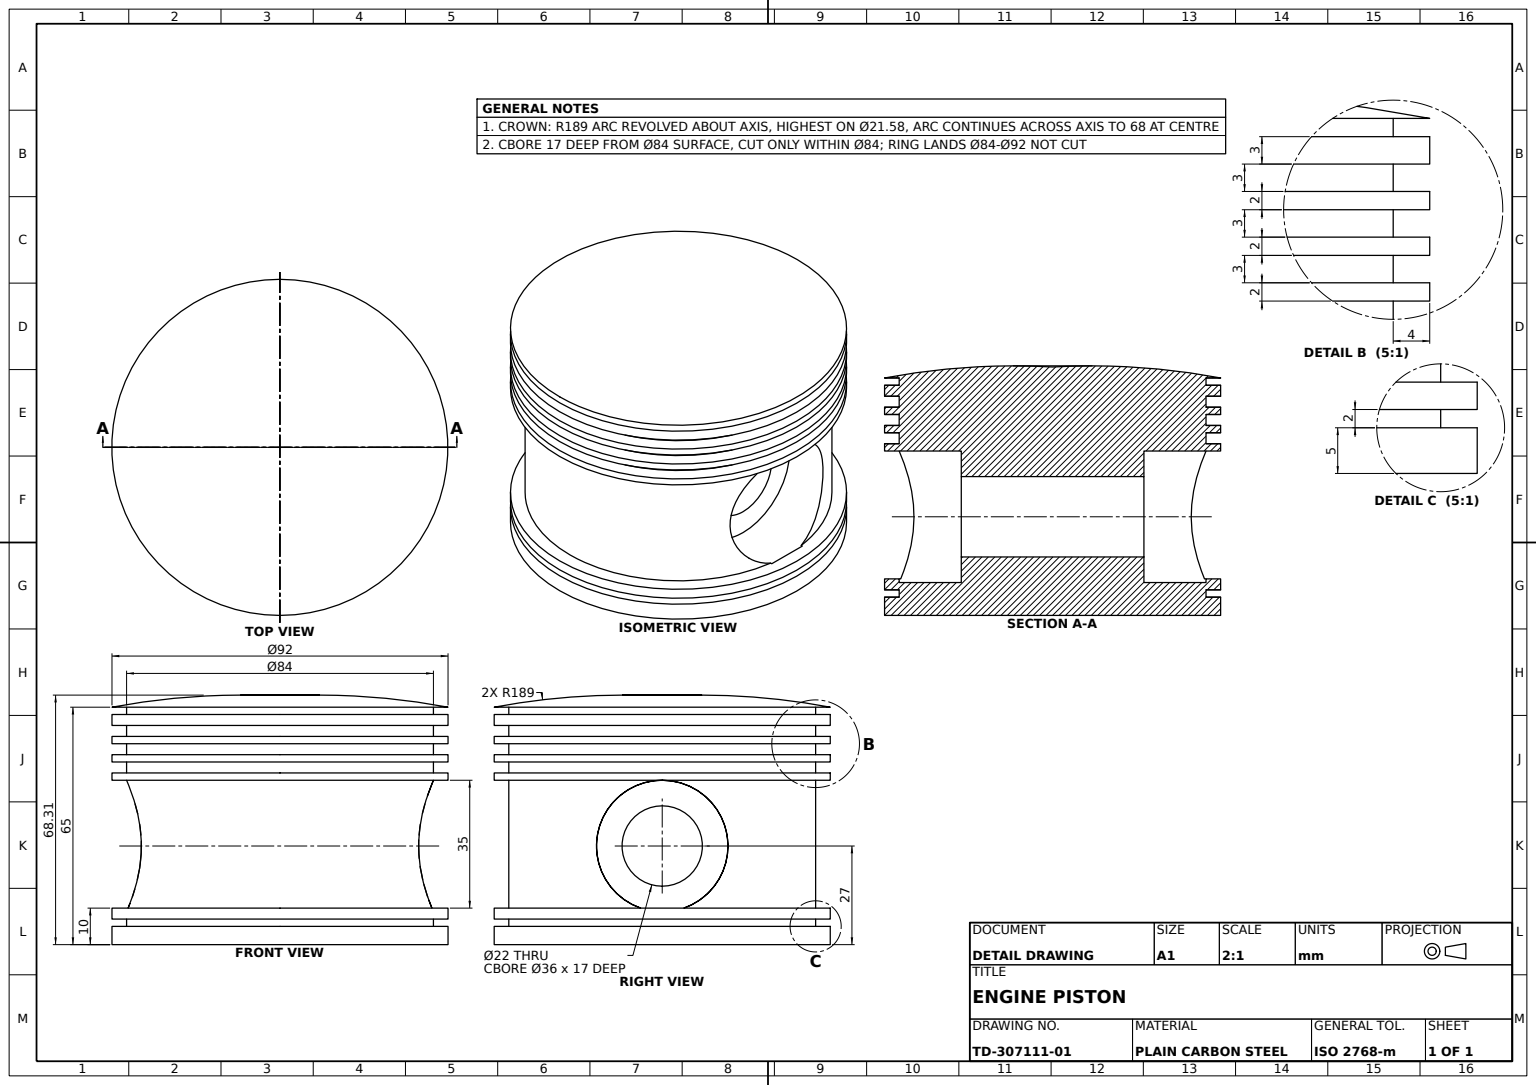
ISO-10303-21;
HEADER;
FILE_DESCRIPTION((''),'2;1');
FILE_NAME('','',(''),(''),'','','');
FILE_SCHEMA(('AUTOMOTIVE_DESIGN'));
ENDSEC;
DATA;
#1=APPLICATION_CONTEXT('');
#2=PRODUCT_CONTEXT('',#1,'mechanical');
#3=PRODUCT('','','',(#2));
#4=PRODUCT_DEFINITION_FORMATION('','',#3);
#5=PRODUCT_DEFINITION_CONTEXT('',#1,'design');
#6=PRODUCT_DEFINITION('','',#4,#5);
#7=PRODUCT_DEFINITION_SHAPE('','',#6);
#8=(LENGTH_UNIT()NAMED_UNIT(*)SI_UNIT(.MILLI.,.METRE.));
#9=(NAMED_UNIT(*)PLANE_ANGLE_UNIT()SI_UNIT($,.RADIAN.));
#10=(NAMED_UNIT(*)SI_UNIT($,.STERADIAN.)SOLID_ANGLE_UNIT());
#11=UNCERTAINTY_MEASURE_WITH_UNIT(LENGTH_MEASURE(1.E-05),#8,'distance_accuracy_value','');
#12=(GEOMETRIC_REPRESENTATION_CONTEXT(3)GLOBAL_UNCERTAINTY_ASSIGNED_CONTEXT((#11))GLOBAL_UNIT_ASSIGNED_CONTEXT((#8,#9,#10))REPRESENTATION_CONTEXT('',''));
#13=CARTESIAN_POINT('',(-46.,0.,-47.));
#14=VERTEX_POINT('',#13);
#15=CARTESIAN_POINT('',(-46.,0.,-45.));
#16=VERTEX_POINT('',#15);
#17=CARTESIAN_POINT('',(-46.,0.,0.));
#18=DIRECTION('',(0.,0.,1.));
#19=VECTOR('',#18,1000.);
#20=LINE('',#17,#19);
#21=EDGE_CURVE('',#14,#16,#20,.T.);
#22=ORIENTED_EDGE('',*,*,#21,.F.);
#23=CARTESIAN_POINT('',(46.,0.,-47.));
#24=VERTEX_POINT('',#23);
#25=CARTESIAN_POINT('',(0.,0.,-47.));
#26=DIRECTION('',(1.,0.,0.));
#27=AXIS2_PLACEMENT_3D('',#25,#18,#26);
#28=CIRCLE('',#27,46.);
#29=EDGE_CURVE('',#14,#24,#28,.T.);
#30=ORIENTED_EDGE('',*,*,#29,.T.);
#31=CARTESIAN_POINT('',(46.,0.,-45.));
#32=VERTEX_POINT('',#31);
#33=CARTESIAN_POINT('',(46.,0.,0.));
#34=LINE('',#33,#19);
#35=EDGE_CURVE('',#24,#32,#34,.T.);
#36=ORIENTED_EDGE('',*,*,#35,.T.);
#37=CARTESIAN_POINT('',(0.,0.,-45.));
#38=AXIS2_PLACEMENT_3D('',#37,#18,#26);
#39=CIRCLE('',#38,46.);
#40=EDGE_CURVE('',#16,#32,#39,.T.);
#41=ORIENTED_EDGE('',*,*,#40,.F.);
#42=EDGE_LOOP('',(#22,#30,#36,#41));
#43=FACE_OUTER_BOUND('',#42,.T.);
#44=CARTESIAN_POINT('',(0.,0.,0.));
#45=AXIS2_PLACEMENT_3D('',#44,#18,#26);
#46=CYLINDRICAL_SURFACE('',#45,46.);
#47=ADVANCED_FACE('',(#43),#46,.T.);
#48=CARTESIAN_POINT('',(46.,0.,-50.));
#49=VERTEX_POINT('',#48);
#50=CARTESIAN_POINT('',(-46.,0.,-50.));
#51=VERTEX_POINT('',#50);
#52=CARTESIAN_POINT('',(0.,0.,-50.));
#53=AXIS2_PLACEMENT_3D('',#52,#18,#26);
#54=CIRCLE('',#53,46.);
#55=EDGE_CURVE('',#49,#51,#54,.T.);
#56=ORIENTED_EDGE('',*,*,#55,.F.);
#57=CARTESIAN_POINT('',(46.,0.,-52.));
#58=VERTEX_POINT('',#57);
#59=EDGE_CURVE('',#58,#49,#34,.T.);
#60=ORIENTED_EDGE('',*,*,#59,.F.);
#61=CARTESIAN_POINT('',(-46.,0.,-52.));
#62=VERTEX_POINT('',#61);
#63=CARTESIAN_POINT('',(0.,0.,-52.));
#64=AXIS2_PLACEMENT_3D('',#63,#18,#26);
#65=CIRCLE('',#64,46.);
#66=EDGE_CURVE('',#58,#62,#65,.T.);
#67=ORIENTED_EDGE('',*,*,#66,.T.);
#68=EDGE_CURVE('',#62,#51,#20,.T.);
#69=ORIENTED_EDGE('',*,*,#68,.T.);
#70=EDGE_LOOP('',(#56,#60,#67,#69));
#71=FACE_OUTER_BOUND('',#70,.T.);
#72=ADVANCED_FACE('',(#71),#46,.T.);
#73=ORIENTED_EDGE('',*,*,#21,.T.);
#74=EDGE_CURVE('',#32,#16,#39,.T.);
#75=ORIENTED_EDGE('',*,*,#74,.F.);
#76=ORIENTED_EDGE('',*,*,#35,.F.);
#77=EDGE_CURVE('',#24,#14,#28,.T.);
#78=ORIENTED_EDGE('',*,*,#77,.T.);
#79=EDGE_LOOP('',(#73,#75,#76,#78));
#80=FACE_OUTER_BOUND('',#79,.T.);
#81=ADVANCED_FACE('',(#80),#46,.T.);
#82=CARTESIAN_POINT('',(42.,0.,-5.));
#83=VERTEX_POINT('',#82);
#84=CARTESIAN_POINT('',(-42.,0.,-5.));
#85=VERTEX_POINT('',#84);
#86=CARTESIAN_POINT('',(0.,0.,-5.));
#87=AXIS2_PLACEMENT_3D('',#86,#18,#26);
#88=CIRCLE('',#87,42.);
#89=EDGE_CURVE('',#83,#85,#88,.T.);
#90=ORIENTED_EDGE('',*,*,#89,.F.);
#91=CARTESIAN_POINT('',(42.,0.,-7.));
#92=VERTEX_POINT('',#91);
#93=CARTESIAN_POINT('',(42.,0.,0.));
#94=LINE('',#93,#19);
#95=EDGE_CURVE('',#92,#83,#94,.T.);
#96=ORIENTED_EDGE('',*,*,#95,.F.);
#97=CARTESIAN_POINT('',(-42.,0.,-7.));
#98=VERTEX_POINT('',#97);
#99=CARTESIAN_POINT('',(0.,0.,-7.));
#100=AXIS2_PLACEMENT_3D('',#99,#18,#26);
#101=CIRCLE('',#100,42.);
#102=EDGE_CURVE('',#92,#98,#101,.T.);
#103=ORIENTED_EDGE('',*,*,#102,.T.);
#104=CARTESIAN_POINT('',(-42.,0.,0.));
#105=LINE('',#104,#19);
#106=EDGE_CURVE('',#98,#85,#105,.T.);
#107=ORIENTED_EDGE('',*,*,#106,.T.);
#108=EDGE_LOOP('',(#90,#96,#103,#107));
#109=FACE_OUTER_BOUND('',#108,.T.);
#110=CYLINDRICAL_SURFACE('',#45,42.);
#111=ADVANCED_FACE('',(#109),#110,.T.);
#112=ORIENTED_EDGE('',*,*,#102,.F.);
#113=EDGE_CURVE('',#98,#92,#101,.T.);
#114=ORIENTED_EDGE('',*,*,#113,.F.);
#115=EDGE_LOOP('',(#112,#114));
#116=FACE_BOUND('',#115,.T.);
#117=CARTESIAN_POINT('',(46.,0.,-7.));
#118=VERTEX_POINT('',#117);
#119=CARTESIAN_POINT('',(-46.,0.,-7.));
#120=VERTEX_POINT('',#119);
#121=CIRCLE('',#100,46.);
#122=EDGE_CURVE('',#118,#120,#121,.T.);
#123=ORIENTED_EDGE('',*,*,#122,.T.);
#124=EDGE_CURVE('',#120,#118,#121,.T.);
#125=ORIENTED_EDGE('',*,*,#124,.T.);
#126=EDGE_LOOP('',(#123,#125));
#127=FACE_OUTER_BOUND('',#126,.T.);
#128=PLANE('',#100);
#129=ADVANCED_FACE('',(#116,#127),#128,.T.);
#130=CARTESIAN_POINT('',(-42.,0.,-55.));
#131=VERTEX_POINT('',#130);
#132=CARTESIAN_POINT('',(42.,0.,-55.));
#133=VERTEX_POINT('',#132);
#134=CARTESIAN_POINT('',(0.,0.,-55.));
#135=AXIS2_PLACEMENT_3D('',#134,#18,#26);
#136=CIRCLE('',#135,42.);
#137=EDGE_CURVE('',#131,#133,#136,.T.);
#138=ORIENTED_EDGE('',*,*,#137,.T.);
#139=CARTESIAN_POINT('',(42.,0.,-52.));
#140=VERTEX_POINT('',#139);
#141=EDGE_CURVE('',#133,#140,#94,.T.);
#142=ORIENTED_EDGE('',*,*,#141,.T.);
#143=CARTESIAN_POINT('',(-42.,0.,-52.));
#144=VERTEX_POINT('',#143);
#145=CIRCLE('',#64,42.);
#146=EDGE_CURVE('',#144,#140,#145,.T.);
#147=ORIENTED_EDGE('',*,*,#146,.F.);
#148=EDGE_CURVE('',#131,#144,#105,.T.);
#149=ORIENTED_EDGE('',*,*,#148,.F.);
#150=EDGE_LOOP('',(#138,#142,#147,#149));
#151=FACE_OUTER_BOUND('',#150,.T.);
#152=ADVANCED_FACE('',(#151),#110,.T.);
#153=CARTESIAN_POINT('',(-5.91608,41.581246,-10.));
#154=VERTEX_POINT('',#153);
#155=CARTESIAN_POINT('',(-5.91608,42.,-10.));
#156=VERTEX_POINT('',#155);
#157=CARTESIAN_POINT('',(-5.91608,25.,-10.));
#158=DIRECTION('',(0.,1.,0.));
#159=VECTOR('',#158,1000.);
#160=LINE('',#157,#159);
#161=EDGE_CURVE('',#154,#156,#160,.T.);
#162=ORIENTED_EDGE('',*,*,#161,.T.);
#163=CARTESIAN_POINT('',(0.,42.,-9.));
#164=VERTEX_POINT('',#163);
#165=CARTESIAN_POINT('',(0.,42.,-27.));
#166=AXIS2_PLACEMENT_3D('',#165,#158,#18);
#167=CIRCLE('',#166,18.);
#168=EDGE_CURVE('',#156,#164,#167,.T.);
#169=ORIENTED_EDGE('',*,*,#168,.T.);
#170=CARTESIAN_POINT('',(0.,25.,-9.));
#171=VERTEX_POINT('',#170);
#172=LINE('',#170,#159);
#173=EDGE_CURVE('',#171,#164,#172,.T.);
#174=ORIENTED_EDGE('',*,*,#173,.F.);
#175=CARTESIAN_POINT('',(0.,25.,-45.));
#176=VERTEX_POINT('',#175);
#177=CARTESIAN_POINT('',(0.,25.,-27.));
#178=AXIS2_PLACEMENT_3D('',#177,#158,#18);
#179=CIRCLE('',#178,18.);
#180=EDGE_CURVE('',#176,#171,#179,.T.);
#181=ORIENTED_EDGE('',*,*,#180,.F.);
#182=CARTESIAN_POINT('',(0.,42.,-45.));
#183=VERTEX_POINT('',#182);
#184=LINE('',#175,#159);
#185=EDGE_CURVE('',#176,#183,#184,.T.);
#186=ORIENTED_EDGE('',*,*,#185,.T.);
#187=CARTESIAN_POINT('',(-1.061109,42.,-45.));
#188=CARTESIAN_POINT('',(-2.121977,41.95976,-44.906731));
#189=CARTESIAN_POINT('',(-4.236491,41.799239,-44.527291));
#190=CARTESIAN_POINT('',(-5.257741,41.68158,-44.24719));
#191=CARTESIAN_POINT('',(-6.739523,41.458754,-43.698988));
#192=CARTESIAN_POINT('',(-7.225049,41.376736,-43.494768));
#193=CARTESIAN_POINT('',(-8.179372,41.198707,-43.042961));
#194=CARTESIAN_POINT('',(-8.64942,41.10235,-42.794419));
#195=CARTESIAN_POINT('',(-10.009425,40.800416,-41.997198));
#196=CARTESIAN_POINT('',(-10.857804,40.580658,-41.394135));
#197=CARTESIAN_POINT('',(-12.047698,40.23709,-40.383712));
#198=CARTESIAN_POINT('',(-12.430461,40.120239,-40.029148));
#199=CARTESIAN_POINT('',(-13.167974,39.884262,-39.283303));
#200=CARTESIAN_POINT('',(-13.519453,39.766169,-38.895167));
#201=CARTESIAN_POINT('',(-14.516037,39.418016,-37.694253));
#202=CARTESIAN_POINT('',(-15.107299,39.192876,-36.841775));
#203=CARTESIAN_POINT('',(-15.885032,38.881149,-35.481657));
#204=CARTESIAN_POINT('',(-16.125966,38.781584,-35.014634));
#205=CARTESIAN_POINT('',(-16.569756,38.594057,-34.051546));
#206=CARTESIAN_POINT('',(-16.769263,38.507524,-33.562673));
#207=CARTESIAN_POINT('',(-17.30133,38.272892,-32.076551));
#208=CARTESIAN_POINT('',(-17.568459,38.149543,-31.058911));
#209=CARTESIAN_POINT('',(-17.83483,38.025366,-29.49002));
#210=CARTESIAN_POINT('',(-17.901168,37.994084,-28.959073));
#211=CARTESIAN_POINT('',(-17.98625,37.95388,-27.885782));
#212=CARTESIAN_POINT('',(-18.004438,37.945227,-27.35139));
#213=CARTESIAN_POINT('',(-17.988399,37.952835,-25.754766));
#214=CARTESIAN_POINT('',(-17.884108,38.002716,-24.699044));
#215=CARTESIAN_POINT('',(-17.586774,38.140757,-23.128397));
#216=CARTESIAN_POINT('',(-17.463221,38.19766,-22.604707));
#217=CARTESIAN_POINT('',(-17.173338,38.328863,-21.581592));
#218=CARTESIAN_POINT('',(-17.00688,38.403227,-21.080313));
#219=CARTESIAN_POINT('',(-16.444866,38.64885,-19.605884));
#220=CARTESIAN_POINT('',(-15.986987,38.842708,-18.661532));
#221=CARTESIAN_POINT('',(-14.902994,39.27137,-16.850389));
#222=CARTESIAN_POINT('',(-14.29136,39.500285,-16.007521));
#223=CARTESIAN_POINT('',(-13.27255,39.84932,-14.830004));
#224=CARTESIAN_POINT('',(-12.915936,39.966639,-14.45207));
#225=CARTESIAN_POINT('',(-12.167816,40.20072,-13.725355));
#226=CARTESIAN_POINT('',(-11.774245,40.318048,-13.374974));
#227=CARTESIAN_POINT('',(-10.556333,40.660487,-12.382869));
#228=CARTESIAN_POINT('',(-9.696644,40.875872,-11.799435));
#229=CARTESIAN_POINT('',(-7.881048,41.264403,-10.783615));
#230=CARTESIAN_POINT('',(-6.925197,41.437671,-10.351177));
#231=B_SPLINE_CURVE_WITH_KNOTS('',3,(#182,#187,#188,#189,#190,#191,#192,#193,#194,#195,#196,#197,#198,#199,#200,#201,#202,#203,#204,#205,#206,#207,#208,#209,#210,#211,#212,#213,#214,#215,#216,#217,#218,#219,#220,#221,#222,#223,#224,#225,#226,#227,#228,#229,#230,#153),.UNSPECIFIED.,.F.,.F.,(4,2,2,2,2,2,2,2,2,2,2,2,2,2,2,2,2,2,2,2,2,2,4),(0.050941496,0.05412348,0.057305464,0.058896456,0.060487448,0.063669432,0.065260424,0.066851416,0.0700334,0.071624392,0.073215384,0.076397368,0.07798836,0.079579352,0.082761336,0.084352328,0.08594332,0.089125304,0.092307288,0.09389828,0.095489272,0.098671256,0.10185324),.UNSPECIFIED.);
#232=EDGE_CURVE('',#183,#154,#231,.T.);
#233=ORIENTED_EDGE('',*,*,#232,.T.);
#234=EDGE_LOOP('',(#162,#169,#174,#181,#186,#233));
#235=FACE_OUTER_BOUND('',#234,.T.);
#236=CYLINDRICAL_SURFACE('',#178,18.);
#237=ADVANCED_FACE('',(#235),#236,.F.);
#238=CARTESIAN_POINT('',(5.91608,42.,-10.));
#239=VERTEX_POINT('',#238);
#240=CARTESIAN_POINT('',(0.,42.,-10.));
#241=VECTOR('',#26,1000.);
#242=LINE('',#240,#241);
#243=EDGE_CURVE('',#156,#239,#242,.T.);
#244=ORIENTED_EDGE('',*,*,#243,.T.);
#245=EDGE_CURVE('',#164,#239,#167,.T.);
#246=ORIENTED_EDGE('',*,*,#245,.F.);
#247=ORIENTED_EDGE('',*,*,#168,.F.);
#248=EDGE_LOOP('',(#244,#246,#247));
#249=FACE_OUTER_BOUND('',#248,.T.);
#250=PLANE('',#166);
#251=ADVANCED_FACE('',(#249),#250,.F.);
#252=ORIENTED_EDGE('',*,*,#77,.F.);
#253=ORIENTED_EDGE('',*,*,#29,.F.);
#254=EDGE_LOOP('',(#252,#253));
#255=FACE_OUTER_BOUND('',#254,.T.);
#256=CARTESIAN_POINT('',(42.,0.,-47.));
#257=VERTEX_POINT('',#256);
#258=CARTESIAN_POINT('',(-42.,0.,-47.));
#259=VERTEX_POINT('',#258);
#260=CIRCLE('',#27,42.);
#261=EDGE_CURVE('',#257,#259,#260,.T.);
#262=ORIENTED_EDGE('',*,*,#261,.T.);
#263=EDGE_CURVE('',#259,#257,#260,.T.);
#264=ORIENTED_EDGE('',*,*,#263,.T.);
#265=EDGE_LOOP('',(#262,#264));
#266=FACE_BOUND('',#265,.T.);
#267=DIRECTION('',(0.,0.,-1.));
#268=DIRECTION('',(-1.,0.,0.));
#269=AXIS2_PLACEMENT_3D('',#25,#267,#268);
#270=PLANE('',#269);
#271=ADVANCED_FACE('',(#255,#266),#270,.T.);
#272=CARTESIAN_POINT('',(-46.,0.,-57.));
#273=VERTEX_POINT('',#272);
#274=CARTESIAN_POINT('',(-46.,0.,-55.));
#275=VERTEX_POINT('',#274);
#276=EDGE_CURVE('',#273,#275,#20,.T.);
#277=ORIENTED_EDGE('',*,*,#276,.T.);
#278=CARTESIAN_POINT('',(46.,0.,-55.));
#279=VERTEX_POINT('',#278);
#280=CIRCLE('',#135,46.);
#281=EDGE_CURVE('',#279,#275,#280,.T.);
#282=ORIENTED_EDGE('',*,*,#281,.F.);
#283=CARTESIAN_POINT('',(46.,0.,-57.));
#284=VERTEX_POINT('',#283);
#285=EDGE_CURVE('',#284,#279,#34,.T.);
#286=ORIENTED_EDGE('',*,*,#285,.F.);
#287=CARTESIAN_POINT('',(0.,0.,-57.));
#288=AXIS2_PLACEMENT_3D('',#287,#18,#26);
#289=CIRCLE('',#288,46.);
#290=EDGE_CURVE('',#284,#273,#289,.T.);
#291=ORIENTED_EDGE('',*,*,#290,.T.);
#292=EDGE_LOOP('',(#277,#282,#286,#291));
#293=FACE_OUTER_BOUND('',#292,.T.);
#294=ADVANCED_FACE('',(#293),#46,.T.);
#295=CARTESIAN_POINT('',(-42.,0.,-50.));
#296=VERTEX_POINT('',#295);
#297=EDGE_CURVE('',#296,#259,#105,.T.);
#298=ORIENTED_EDGE('',*,*,#297,.T.);
#299=ORIENTED_EDGE('',*,*,#261,.F.);
#300=CARTESIAN_POINT('',(42.,0.,-50.));
#301=VERTEX_POINT('',#300);
#302=EDGE_CURVE('',#301,#257,#94,.T.);
#303=ORIENTED_EDGE('',*,*,#302,.F.);
#304=CIRCLE('',#53,42.);
#305=EDGE_CURVE('',#301,#296,#304,.T.);
#306=ORIENTED_EDGE('',*,*,#305,.T.);
#307=EDGE_LOOP('',(#298,#299,#303,#306));
#308=FACE_OUTER_BOUND('',#307,.T.);
#309=ADVANCED_FACE('',(#308),#110,.T.);
#310=ORIENTED_EDGE('',*,*,#180,.T.);
#311=EDGE_CURVE('',#171,#176,#179,.T.);
#312=ORIENTED_EDGE('',*,*,#311,.T.);
#313=EDGE_LOOP('',(#310,#312));
#314=FACE_OUTER_BOUND('',#313,.T.);
#315=CARTESIAN_POINT('',(0.,25.,-16.));
#316=VERTEX_POINT('',#315);
#317=CARTESIAN_POINT('',(0.,25.,-38.));
#318=VERTEX_POINT('',#317);
#319=CIRCLE('',#178,11.);
#320=EDGE_CURVE('',#316,#318,#319,.T.);
#321=ORIENTED_EDGE('',*,*,#320,.F.);
#322=EDGE_CURVE('',#318,#316,#319,.T.);
#323=ORIENTED_EDGE('',*,*,#322,.F.);
#324=EDGE_LOOP('',(#321,#323));
#325=FACE_BOUND('',#324,.T.);
#326=PLANE('',#178);
#327=ADVANCED_FACE('',(#314,#325),#326,.T.);
#328=EDGE_CURVE('',#275,#279,#280,.T.);
#329=ORIENTED_EDGE('',*,*,#328,.F.);
#330=ORIENTED_EDGE('',*,*,#276,.F.);
#331=EDGE_CURVE('',#273,#284,#289,.T.);
#332=ORIENTED_EDGE('',*,*,#331,.T.);
#333=ORIENTED_EDGE('',*,*,#285,.T.);
#334=EDGE_LOOP('',(#329,#330,#332,#333));
#335=FACE_OUTER_BOUND('',#334,.T.);
#336=ADVANCED_FACE('',(#335),#46,.T.);
#337=CARTESIAN_POINT('',(-46.,0.,-5.));
#338=VERTEX_POINT('',#337);
#339=VERTEX_POINT('',#17);
#340=EDGE_CURVE('',#338,#339,#20,.T.);
#341=ORIENTED_EDGE('',*,*,#340,.F.);
#342=CARTESIAN_POINT('',(46.,0.,-5.));
#343=VERTEX_POINT('',#342);
#344=CIRCLE('',#87,46.);
#345=EDGE_CURVE('',#338,#343,#344,.T.);
#346=ORIENTED_EDGE('',*,*,#345,.T.);
#347=VERTEX_POINT('',#33);
#348=EDGE_CURVE('',#343,#347,#34,.T.);
#349=ORIENTED_EDGE('',*,*,#348,.T.);
#350=CIRCLE('',#45,46.);
#351=EDGE_CURVE('',#339,#347,#350,.T.);
#352=ORIENTED_EDGE('',*,*,#351,.F.);
#353=EDGE_LOOP('',(#341,#346,#349,#352));
#354=FACE_OUTER_BOUND('',#353,.T.);
#355=ADVANCED_FACE('',(#354),#46,.T.);
#356=EDGE_CURVE('',#51,#49,#54,.T.);
#357=ORIENTED_EDGE('',*,*,#356,.F.);
#358=ORIENTED_EDGE('',*,*,#68,.F.);
#359=EDGE_CURVE('',#62,#58,#65,.T.);
#360=ORIENTED_EDGE('',*,*,#359,.T.);
#361=ORIENTED_EDGE('',*,*,#59,.T.);
#362=EDGE_LOOP('',(#357,#358,#360,#361));
#363=FACE_OUTER_BOUND('',#362,.T.);
#364=ADVANCED_FACE('',(#363),#46,.T.);
#365=CARTESIAN_POINT('',(46.,0.,-10.));
#366=VERTEX_POINT('',#365);
#367=CARTESIAN_POINT('',(-46.,0.,-10.));
#368=VERTEX_POINT('',#367);
#369=CARTESIAN_POINT('',(0.,0.,-10.));
#370=AXIS2_PLACEMENT_3D('',#369,#18,#26);
#371=CIRCLE('',#370,46.);
#372=EDGE_CURVE('',#366,#368,#371,.T.);
#373=ORIENTED_EDGE('',*,*,#372,.F.);
#374=EDGE_CURVE('',#368,#366,#371,.T.);
#375=ORIENTED_EDGE('',*,*,#374,.F.);
#376=EDGE_LOOP('',(#373,#375));
#377=FACE_OUTER_BOUND('',#376,.T.);
#378=CARTESIAN_POINT('',(42.,0.,-10.));
#379=VERTEX_POINT('',#378);
#380=CARTESIAN_POINT('',(5.91608,41.581246,-10.));
#381=VERTEX_POINT('',#380);
#382=CIRCLE('',#370,42.);
#383=EDGE_CURVE('',#379,#381,#382,.T.);
#384=ORIENTED_EDGE('',*,*,#383,.T.);
#385=CARTESIAN_POINT('',(5.91608,25.,-10.));
#386=DIRECTION('',(0.,-1.,0.));
#387=VECTOR('',#386,1000.);
#388=LINE('',#385,#387);
#389=EDGE_CURVE('',#239,#381,#388,.T.);
#390=ORIENTED_EDGE('',*,*,#389,.F.);
#391=ORIENTED_EDGE('',*,*,#243,.F.);
#392=ORIENTED_EDGE('',*,*,#161,.F.);
#393=CARTESIAN_POINT('',(-5.91608,-41.581246,-10.));
#394=VERTEX_POINT('',#393);
#395=EDGE_CURVE('',#154,#394,#382,.T.);
#396=ORIENTED_EDGE('',*,*,#395,.T.);
#397=CARTESIAN_POINT('',(-5.91608,-42.,-10.));
#398=VERTEX_POINT('',#397);
#399=CARTESIAN_POINT('',(-5.91608,-25.,-10.));
#400=LINE('',#399,#387);
#401=EDGE_CURVE('',#394,#398,#400,.T.);
#402=ORIENTED_EDGE('',*,*,#401,.T.);
#403=CARTESIAN_POINT('',(5.91608,-42.,-10.));
#404=VERTEX_POINT('',#403);
#405=CARTESIAN_POINT('',(0.,-42.,-10.));
#406=VECTOR('',#268,1000.);
#407=LINE('',#405,#406);
#408=EDGE_CURVE('',#404,#398,#407,.T.);
#409=ORIENTED_EDGE('',*,*,#408,.F.);
#410=CARTESIAN_POINT('',(5.91608,-41.581246,-10.));
#411=VERTEX_POINT('',#410);
#412=CARTESIAN_POINT('',(5.91608,-25.,-10.));
#413=LINE('',#412,#159);
#414=EDGE_CURVE('',#404,#411,#413,.T.);
#415=ORIENTED_EDGE('',*,*,#414,.T.);
#416=EDGE_CURVE('',#411,#379,#382,.T.);
#417=ORIENTED_EDGE('',*,*,#416,.T.);
#418=EDGE_LOOP('',(#384,#390,#391,#392,#396,#402,#409,#415,#417));
#419=FACE_BOUND('',#418,.T.);
#420=AXIS2_PLACEMENT_3D('',#369,#267,#268);
#421=PLANE('',#420);
#422=ADVANCED_FACE('',(#377,#419),#421,.T.);
#423=CARTESIAN_POINT('',(-46.,0.,-60.));
#424=VERTEX_POINT('',#423);
#425=CARTESIAN_POINT('',(46.,0.,-60.));
#426=VERTEX_POINT('',#425);
#427=CARTESIAN_POINT('',(0.,0.,-60.));
#428=AXIS2_PLACEMENT_3D('',#427,#18,#26);
#429=CIRCLE('',#428,46.);
#430=EDGE_CURVE('',#424,#426,#429,.T.);
#431=ORIENTED_EDGE('',*,*,#430,.F.);
#432=CARTESIAN_POINT('',(-46.,0.,-63.));
#433=VERTEX_POINT('',#432);
#434=EDGE_CURVE('',#433,#424,#20,.T.);
#435=ORIENTED_EDGE('',*,*,#434,.F.);
#436=CARTESIAN_POINT('',(46.,0.,-63.));
#437=VERTEX_POINT('',#436);
#438=CARTESIAN_POINT('',(0.,0.,-63.));
#439=AXIS2_PLACEMENT_3D('',#438,#18,#26);
#440=CIRCLE('',#439,46.);
#441=EDGE_CURVE('',#433,#437,#440,.T.);
#442=ORIENTED_EDGE('',*,*,#441,.T.);
#443=EDGE_CURVE('',#437,#426,#34,.T.);
#444=ORIENTED_EDGE('',*,*,#443,.T.);
#445=EDGE_LOOP('',(#431,#435,#442,#444));
#446=FACE_OUTER_BOUND('',#445,.T.);
#447=ADVANCED_FACE('',(#446),#46,.T.);
#448=CARTESIAN_POINT('',(42.,0.,-57.));
#449=VERTEX_POINT('',#448);
#450=CARTESIAN_POINT('',(-42.,0.,-57.));
#451=VERTEX_POINT('',#450);
#452=CIRCLE('',#288,42.);
#453=EDGE_CURVE('',#449,#451,#452,.T.);
#454=ORIENTED_EDGE('',*,*,#453,.T.);
#455=EDGE_CURVE('',#451,#449,#452,.T.);
#456=ORIENTED_EDGE('',*,*,#455,.T.);
#457=EDGE_LOOP('',(#454,#456));
#458=FACE_BOUND('',#457,.T.);
#459=ORIENTED_EDGE('',*,*,#290,.F.);
#460=ORIENTED_EDGE('',*,*,#331,.F.);
#461=EDGE_LOOP('',(#459,#460));
#462=FACE_OUTER_BOUND('',#461,.T.);
#463=AXIS2_PLACEMENT_3D('',#287,#267,#268);
#464=PLANE('',#463);
#465=ADVANCED_FACE('',(#458,#462),#464,.T.);
#466=CARTESIAN_POINT('',(-46.,0.,-65.));
#467=VERTEX_POINT('',#466);
#468=CARTESIAN_POINT('',(46.,0.,-65.));
#469=VERTEX_POINT('',#468);
#470=CARTESIAN_POINT('',(0.,0.,-65.));
#471=AXIS2_PLACEMENT_3D('',#470,#18,#26);
#472=CIRCLE('',#471,46.);
#473=EDGE_CURVE('',#467,#469,#472,.T.);
#474=ORIENTED_EDGE('',*,*,#473,.F.);
#475=CARTESIAN_POINT('',(0.,0.,-68.));
#476=VERTEX_POINT('',#475);
#477=CARTESIAN_POINT('',(-10.791849,0.,120.691643));
#478=AXIS2_PLACEMENT_3D('',#477,#158,#268);
#479=CIRCLE('',#478,189.);
#480=EDGE_CURVE('',#476,#467,#479,.T.);
#481=ORIENTED_EDGE('',*,*,#480,.F.);
#482=CARTESIAN_POINT('',(10.791849,0.,120.691643));
#483=AXIS2_PLACEMENT_3D('',#482,#386,#267);
#484=CIRCLE('',#483,189.);
#485=EDGE_CURVE('',#476,#469,#484,.T.);
#486=ORIENTED_EDGE('',*,*,#485,.T.);
#487=EDGE_LOOP('',(#474,#481,#486));
#488=FACE_OUTER_BOUND('',#487,.T.);
#489=CARTESIAN_POINT('',(0.,0.,120.691643));
#490=AXIS2_PLACEMENT_3D('',#489,#18,#26);
#491=TOROIDAL_SURFACE('',#490,10.791849,189.);
#492=ADVANCED_FACE('',(#488),#491,.T.);
#493=ORIENTED_EDGE('',*,*,#141,.F.);
#494=EDGE_CURVE('',#133,#131,#136,.T.);
#495=ORIENTED_EDGE('',*,*,#494,.T.);
#496=ORIENTED_EDGE('',*,*,#148,.T.);
#497=EDGE_CURVE('',#140,#144,#145,.T.);
#498=ORIENTED_EDGE('',*,*,#497,.F.);
#499=EDGE_LOOP('',(#493,#495,#496,#498));
#500=FACE_OUTER_BOUND('',#499,.T.);
#501=ADVANCED_FACE('',(#500),#110,.T.);
#502=CARTESIAN_POINT('',(42.,0.,-60.));
#503=VERTEX_POINT('',#502);
#504=CARTESIAN_POINT('',(-42.,0.,-60.));
#505=VERTEX_POINT('',#504);
#506=CIRCLE('',#428,42.);
#507=EDGE_CURVE('',#503,#505,#506,.T.);
#508=ORIENTED_EDGE('',*,*,#507,.F.);
#509=EDGE_CURVE('',#505,#503,#506,.T.);
#510=ORIENTED_EDGE('',*,*,#509,.F.);
#511=EDGE_LOOP('',(#508,#510));
#512=FACE_BOUND('',#511,.T.);
#513=EDGE_CURVE('',#426,#424,#429,.T.);
#514=ORIENTED_EDGE('',*,*,#513,.T.);
#515=ORIENTED_EDGE('',*,*,#430,.T.);
#516=EDGE_LOOP('',(#514,#515));
#517=FACE_OUTER_BOUND('',#516,.T.);
#518=PLANE('',#428);
#519=ADVANCED_FACE('',(#512,#517),#518,.T.);
#520=EDGE_CURVE('',#368,#120,#20,.T.);
#521=ORIENTED_EDGE('',*,*,#520,.T.);
#522=ORIENTED_EDGE('',*,*,#122,.F.);
#523=EDGE_CURVE('',#366,#118,#34,.T.);
#524=ORIENTED_EDGE('',*,*,#523,.F.);
#525=ORIENTED_EDGE('',*,*,#372,.T.);
#526=EDGE_LOOP('',(#521,#522,#524,#525));
#527=FACE_OUTER_BOUND('',#526,.T.);
#528=ADVANCED_FACE('',(#527),#46,.T.);
#529=ORIENTED_EDGE('',*,*,#389,.T.);
#530=CARTESIAN_POINT('',(6.92465,41.437749,-10.350987));
#531=CARTESIAN_POINT('',(7.881826,41.264313,-10.783798));
#532=CARTESIAN_POINT('',(9.247335,40.971984,-11.548175));
#533=CARTESIAN_POINT('',(9.690715,40.869156,-11.822299));
#534=CARTESIAN_POINT('',(10.554151,40.654739,-12.409507));
#535=CARTESIAN_POINT('',(10.975418,40.542801,-12.723591));
#536=CARTESIAN_POINT('',(12.195632,40.199263,-13.719593));
#537=CARTESIAN_POINT('',(12.93925,39.963601,-14.444107));
#538=CARTESIAN_POINT('',(13.956173,39.615068,-15.620461));
#539=CARTESIAN_POINT('',(14.278615,39.499715,-16.027611));
#540=CARTESIAN_POINT('',(14.890143,39.273273,-16.873016));
#541=CARTESIAN_POINT('',(15.180498,39.161672,-17.313478));
#542=CARTESIAN_POINT('',(15.989482,38.841638,-18.666851));
#543=CARTESIAN_POINT('',(16.445018,38.648769,-19.606851));
#544=CARTESIAN_POINT('',(17.004942,38.404081,-21.074947));
#545=CARTESIAN_POINT('',(17.170887,38.32996,-21.57405));
#546=CARTESIAN_POINT('',(17.460121,38.199076,-22.592677));
#547=CARTESIAN_POINT('',(17.583935,38.142068,-23.115294));
#548=CARTESIAN_POINT('',(17.883221,38.003142,-24.690632));
#549=CARTESIAN_POINT('',(17.987617,37.953205,-25.746325));
#550=CARTESIAN_POINT('',(18.004646,37.945128,-27.337976));
#551=CARTESIAN_POINT('',(17.986924,37.95356,-27.869885));
#552=CARTESIAN_POINT('',(17.903524,37.992972,-28.936481));
#553=CARTESIAN_POINT('',(17.837309,38.024203,-29.472858));
#554=CARTESIAN_POINT('',(17.570657,38.148532,-31.050988));
#555=CARTESIAN_POINT('',(17.302563,38.272346,-32.072983));
#556=CARTESIAN_POINT('',(16.769013,38.507635,-33.563433));
#557=CARTESIAN_POINT('',(16.568539,38.594578,-34.054367));
#558=CARTESIAN_POINT('',(16.12504,38.781968,-35.016462));
#559=CARTESIAN_POINT('',(15.884064,38.881547,-35.483504));
#560=CARTESIAN_POINT('',(15.105336,39.193643,-36.844901));
#561=CARTESIAN_POINT('',(14.512273,39.419472,-37.699857));
#562=CARTESIAN_POINT('',(13.510018,39.769393,-38.905993));
#563=CARTESIAN_POINT('',(13.15582,39.888257,-39.29621));
#564=CARTESIAN_POINT('',(12.421279,40.123067,-40.0378));
#565=CARTESIAN_POINT('',(12.039734,40.239464,-40.390823));
#566=CARTESIAN_POINT('',(10.852425,40.58206,-41.397995));
#567=CARTESIAN_POINT('',(10.004365,40.801702,-42.000713));
#568=CARTESIAN_POINT('',(8.641433,41.104041,-42.798823));
#569=CARTESIAN_POINT('',(8.171271,41.200301,-43.047045));
#570=CARTESIAN_POINT('',(7.219154,41.377752,-43.497307));
#571=CARTESIAN_POINT('',(6.734881,41.459491,-43.700811));
#572=CARTESIAN_POINT('',(5.257349,41.68156,-44.247121));
#573=CARTESIAN_POINT('',(4.239576,41.798818,-44.526284));
#574=CARTESIAN_POINT('',(2.660115,41.919,-44.810389));
#575=CARTESIAN_POINT('',(2.125152,41.949573,-44.882072));
#576=CARTESIAN_POINT('',(1.062066,41.989939,-44.976562));
#577=CARTESIAN_POINT('',(0.530864,42.,-45.));
#578=B_SPLINE_CURVE_WITH_KNOTS('',3,(#380,#530,#531,#532,#533,#534,#535,#536,#537,#538,#539,#540,#541,#542,#543,#544,#545,#546,#547,#548,#549,#550,#551,#552,#553,#554,#555,#556,#557,#558,#559,#560,#561,#562,#563,#564,#565,#566,#567,#568,#569,#570,#571,#572,#573,#574,#575,#576,#577,#182),.UNSPECIFIED.,.F.,.F.,(4,2,2,2,2,2,2,2,2,2,2,2,2,2,2,2,2,2,2,2,2,2,2,2,4),(0.,0.003183844,0.004775765,0.006367687,0.009551531,0.011143452,0.012735374,0.015919218,0.017511139,0.019103061,0.022286905,0.023878826,0.025470748,0.028654592,0.030246513,0.031838435,0.035022279,0.0366142,0.038206122,0.041389966,0.042981887,0.044573809,0.047757653,0.049349574,0.050941496),.UNSPECIFIED.);
#579=EDGE_CURVE('',#381,#183,#578,.T.);
#580=ORIENTED_EDGE('',*,*,#579,.T.);
#581=ORIENTED_EDGE('',*,*,#185,.F.);
#582=ORIENTED_EDGE('',*,*,#311,.F.);
#583=ORIENTED_EDGE('',*,*,#173,.T.);
#584=ORIENTED_EDGE('',*,*,#245,.T.);
#585=EDGE_LOOP('',(#529,#580,#581,#582,#583,#584));
#586=FACE_OUTER_BOUND('',#585,.T.);
#587=ADVANCED_FACE('',(#586),#236,.F.);
#588=CARTESIAN_POINT('',(42.,0.,-45.));
#589=VERTEX_POINT('',#588);
#590=EDGE_CURVE('',#589,#379,#94,.T.);
#591=ORIENTED_EDGE('',*,*,#590,.F.);
#592=CIRCLE('',#38,42.);
#593=EDGE_CURVE('',#589,#183,#592,.T.);
#594=ORIENTED_EDGE('',*,*,#593,.T.);
#595=ORIENTED_EDGE('',*,*,#579,.F.);
#596=ORIENTED_EDGE('',*,*,#383,.F.);
#597=EDGE_LOOP('',(#591,#594,#595,#596));
#598=FACE_OUTER_BOUND('',#597,.T.);
#599=ADVANCED_FACE('',(#598),#110,.T.);
#600=ORIENTED_EDGE('',*,*,#494,.F.);
#601=ORIENTED_EDGE('',*,*,#137,.F.);
#602=EDGE_LOOP('',(#600,#601));
#603=FACE_BOUND('',#602,.T.);
#604=ORIENTED_EDGE('',*,*,#281,.T.);
#605=ORIENTED_EDGE('',*,*,#328,.T.);
#606=EDGE_LOOP('',(#604,#605));
#607=FACE_OUTER_BOUND('',#606,.T.);
#608=PLANE('',#135);
#609=ADVANCED_FACE('',(#603,#607),#608,.T.);
#610=CARTESIAN_POINT('',(0.,-25.,-45.));
#611=VERTEX_POINT('',#610);
#612=CARTESIAN_POINT('',(0.,-25.,-9.));
#613=VERTEX_POINT('',#612);
#614=CARTESIAN_POINT('',(0.,-25.,-27.));
#615=AXIS2_PLACEMENT_3D('',#614,#158,#18);
#616=CIRCLE('',#615,18.);
#617=EDGE_CURVE('',#611,#613,#616,.T.);
#618=ORIENTED_EDGE('',*,*,#617,.T.);
#619=CARTESIAN_POINT('',(0.,-42.,-9.));
#620=VERTEX_POINT('',#619);
#621=LINE('',#612,#387);
#622=EDGE_CURVE('',#613,#620,#621,.T.);
#623=ORIENTED_EDGE('',*,*,#622,.T.);
#624=CARTESIAN_POINT('',(0.,-42.,-27.));
#625=AXIS2_PLACEMENT_3D('',#624,#158,#18);
#626=CIRCLE('',#625,18.);
#627=EDGE_CURVE('',#398,#620,#626,.T.);
#628=ORIENTED_EDGE('',*,*,#627,.F.);
#629=ORIENTED_EDGE('',*,*,#401,.F.);
#630=CARTESIAN_POINT('',(0.,-42.,-45.));
#631=VERTEX_POINT('',#630);
#632=CARTESIAN_POINT('',(-1.07712,-42.,-45.));
#633=CARTESIAN_POINT('',(-2.135947,-41.958657,-44.90412));
#634=CARTESIAN_POINT('',(-3.698323,-41.840115,-44.623914));
#635=CARTESIAN_POINT('',(-4.214779,-41.791162,-44.507636));
#636=CARTESIAN_POINT('',(-5.239002,-41.675154,-44.228887));
#637=CARTESIAN_POINT('',(-5.749282,-41.607676,-44.065373));
#638=CARTESIAN_POINT('',(-7.241261,-41.38328,-43.513296));
#639=CARTESIAN_POINT('',(-8.187959,-41.204499,-43.063911));
#640=CARTESIAN_POINT('',(-9.540827,-40.904596,-42.27238));
#641=CARTESIAN_POINT('',(-9.980516,-40.799324,-41.988831));
#642=CARTESIAN_POINT('',(-10.837334,-40.58014,-41.381514));
#643=CARTESIAN_POINT('',(-11.252743,-40.466611,-41.058703));
#644=CARTESIAN_POINT('',(-12.444045,-40.122675,-40.047267));
#645=CARTESIAN_POINT('',(-13.172573,-39.88708,-39.311131));
#646=CARTESIAN_POINT('',(-14.502239,-39.423101,-37.712874));
#647=CARTESIAN_POINT('',(-15.106289,-39.193257,-36.843177));
#648=CARTESIAN_POINT('',(-16.142197,-38.778097,-35.032284));
#649=CARTESIAN_POINT('',(-16.580004,-38.590867,-34.085912));
#650=CARTESIAN_POINT('',(-17.114425,-38.355369,-32.601172));
#651=CARTESIAN_POINT('',(-17.272128,-38.284408,-32.095057));
#652=CARTESIAN_POINT('',(-17.544158,-38.160514,-31.060609));
#653=CARTESIAN_POINT('',(-17.656264,-38.108607,-30.54078));
#654=CARTESIAN_POINT('',(-17.922836,-37.984344,-28.973602));
#655=CARTESIAN_POINT('',(-18.008094,-37.943493,-27.91861));
#656=CARTESIAN_POINT('',(-17.995055,-37.949678,-26.320419));
#657=CARTESIAN_POINT('',(-17.966763,-37.963123,-25.782213));
#658=CARTESIAN_POINT('',(-17.862398,-38.012341,-24.714755));
#659=CARTESIAN_POINT('',(-17.786836,-38.047867,-24.187653));
#660=CARTESIAN_POINT('',(-17.492453,-38.184564,-22.625374));
#661=CARTESIAN_POINT('',(-17.206483,-38.315864,-21.609101));
#662=CARTESIAN_POINT('',(-16.642374,-38.562592,-20.121585));
#663=CARTESIAN_POINT('',(-16.43211,-38.652907,-19.633754));
#664=CARTESIAN_POINT('',(-15.974659,-38.844198,-18.688195));
#665=CARTESIAN_POINT('',(-15.726656,-38.945535,-18.228229));
#666=CARTESIAN_POINT('',(-15.192733,-39.156906,-17.332916));
#667=CARTESIAN_POINT('',(-14.906813,-39.266943,-16.89757));
#668=CARTESIAN_POINT('',(-14.296666,-39.493179,-16.05114));
#669=CARTESIAN_POINT('',(-13.971011,-39.609867,-15.638448));
#670=CARTESIAN_POINT('',(-12.945208,-39.961786,-14.449396));
#671=CARTESIAN_POINT('',(-12.201714,-40.197193,-13.726159));
#672=CARTESIAN_POINT('',(-10.997117,-40.536865,-12.740527));
#673=CARTESIAN_POINT('',(-10.580597,-40.647869,-12.428636));
#674=CARTESIAN_POINT('',(-9.716427,-40.863056,-11.838709));
#675=CARTESIAN_POINT('',(-9.266878,-40.967626,-11.559687));
#676=CARTESIAN_POINT('',(-7.886644,-41.263622,-10.785377));
#677=CARTESIAN_POINT('',(-6.923915,-41.437853,-10.350732));
#678=B_SPLINE_CURVE_WITH_KNOTS('',3,(#630,#632,#633,#634,#635,#636,#637,#638,#639,#640,#641,#642,#643,#644,#645,#646,#647,#648,#649,#650,#651,#652,#653,#654,#655,#656,#657,#658,#659,#660,#661,#662,#663,#664,#665,#666,#667,#668,#669,#670,#671,#672,#673,#674,#675,#676,#677,#393),.UNSPECIFIED.,.F.,.F.,(4,2,2,2,2,2,2,2,2,2,2,2,2,2,2,2,2,2,2,2,2,2,2,4),(0.,0.003182879,0.004774319,0.006365759,0.009548638,0.011140078,0.012731517,0.015914397,0.019097276,0.022280156,0.023871595,0.025463035,0.028645914,0.030237354,0.031828794,0.035011673,0.036603113,0.038194552,0.039785992,0.041377432,0.044560311,0.046151751,0.04774319,0.05092607),.UNSPECIFIED.);
#679=EDGE_CURVE('',#631,#394,#678,.T.);
#680=ORIENTED_EDGE('',*,*,#679,.F.);
#681=LINE('',#610,#387);
#682=EDGE_CURVE('',#611,#631,#681,.T.);
#683=ORIENTED_EDGE('',*,*,#682,.F.);
#684=EDGE_LOOP('',(#618,#623,#628,#629,#680,#683));
#685=FACE_OUTER_BOUND('',#684,.T.);
#686=AXIS2_PLACEMENT_3D('',#614,#386,#267);
#687=CYLINDRICAL_SURFACE('',#686,18.);
#688=ADVANCED_FACE('',(#685),#687,.F.);
#689=ORIENTED_EDGE('',*,*,#95,.T.);
#690=EDGE_CURVE('',#85,#83,#88,.T.);
#691=ORIENTED_EDGE('',*,*,#690,.F.);
#692=ORIENTED_EDGE('',*,*,#106,.F.);
#693=ORIENTED_EDGE('',*,*,#113,.T.);
#694=EDGE_LOOP('',(#689,#691,#692,#693));
#695=FACE_OUTER_BOUND('',#694,.T.);
#696=ADVANCED_FACE('',(#695),#110,.T.);
#697=ORIENTED_EDGE('',*,*,#124,.F.);
#698=ORIENTED_EDGE('',*,*,#520,.F.);
#699=ORIENTED_EDGE('',*,*,#374,.T.);
#700=ORIENTED_EDGE('',*,*,#523,.T.);
#701=EDGE_LOOP('',(#697,#698,#699,#700));
#702=FACE_OUTER_BOUND('',#701,.T.);
#703=ADVANCED_FACE('',(#702),#46,.T.);
#704=EDGE_CURVE('',#505,#451,#105,.T.);
#705=ORIENTED_EDGE('',*,*,#704,.F.);
#706=ORIENTED_EDGE('',*,*,#509,.T.);
#707=EDGE_CURVE('',#503,#449,#94,.T.);
#708=ORIENTED_EDGE('',*,*,#707,.T.);
#709=ORIENTED_EDGE('',*,*,#455,.F.);
#710=EDGE_LOOP('',(#705,#706,#708,#709));
#711=FACE_OUTER_BOUND('',#710,.T.);
#712=ADVANCED_FACE('',(#711),#110,.T.);
#713=ORIENTED_EDGE('',*,*,#453,.F.);
#714=ORIENTED_EDGE('',*,*,#707,.F.);
#715=ORIENTED_EDGE('',*,*,#507,.T.);
#716=ORIENTED_EDGE('',*,*,#704,.T.);
#717=EDGE_LOOP('',(#713,#714,#715,#716));
#718=FACE_OUTER_BOUND('',#717,.T.);
#719=ADVANCED_FACE('',(#718),#110,.T.);
#720=ORIENTED_EDGE('',*,*,#74,.T.);
#721=ORIENTED_EDGE('',*,*,#40,.T.);
#722=EDGE_LOOP('',(#720,#721));
#723=FACE_OUTER_BOUND('',#722,.T.);
#724=ORIENTED_EDGE('',*,*,#593,.F.);
#725=EDGE_CURVE('',#631,#589,#592,.T.);
#726=ORIENTED_EDGE('',*,*,#725,.F.);
#727=EDGE_CURVE('',#183,#631,#592,.T.);
#728=ORIENTED_EDGE('',*,*,#727,.F.);
#729=EDGE_LOOP('',(#724,#726,#728));
#730=FACE_BOUND('',#729,.T.);
#731=PLANE('',#38);
#732=ADVANCED_FACE('',(#723,#730),#731,.T.);
#733=EDGE_CURVE('',#296,#301,#304,.T.);
#734=ORIENTED_EDGE('',*,*,#733,.F.);
#735=ORIENTED_EDGE('',*,*,#305,.F.);
#736=EDGE_LOOP('',(#734,#735));
#737=FACE_BOUND('',#736,.T.);
#738=ORIENTED_EDGE('',*,*,#356,.T.);
#739=ORIENTED_EDGE('',*,*,#55,.T.);
#740=EDGE_LOOP('',(#738,#739));
#741=FACE_OUTER_BOUND('',#740,.T.);
#742=PLANE('',#53);
#743=ADVANCED_FACE('',(#737,#741),#742,.T.);
#744=CARTESIAN_POINT('',(0.,-25.,-16.));
#745=VERTEX_POINT('',#744);
#746=CARTESIAN_POINT('',(0.,-132.,-16.));
#747=LINE('',#746,#159);
#748=EDGE_CURVE('',#745,#316,#747,.T.);
#749=ORIENTED_EDGE('',*,*,#748,.T.);
#750=ORIENTED_EDGE('',*,*,#320,.T.);
#751=CARTESIAN_POINT('',(0.,-25.,-38.));
#752=VERTEX_POINT('',#751);
#753=CARTESIAN_POINT('',(0.,-132.,-38.));
#754=LINE('',#753,#159);
#755=EDGE_CURVE('',#752,#318,#754,.T.);
#756=ORIENTED_EDGE('',*,*,#755,.F.);
#757=CIRCLE('',#686,11.);
#758=EDGE_CURVE('',#752,#745,#757,.T.);
#759=ORIENTED_EDGE('',*,*,#758,.T.);
#760=EDGE_LOOP('',(#749,#750,#756,#759));
#761=FACE_OUTER_BOUND('',#760,.T.);
#762=CARTESIAN_POINT('',(0.,-132.,-27.));
#763=AXIS2_PLACEMENT_3D('',#762,#158,#18);
#764=CYLINDRICAL_SURFACE('',#763,11.);
#765=ADVANCED_FACE('',(#761),#764,.F.);
#766=EDGE_CURVE('',#347,#339,#350,.T.);
#767=ORIENTED_EDGE('',*,*,#766,.T.);
#768=ORIENTED_EDGE('',*,*,#351,.T.);
#769=EDGE_LOOP('',(#767,#768));
#770=FACE_OUTER_BOUND('',#769,.T.);
#771=PLANE('',#45);
#772=ADVANCED_FACE('',(#770),#771,.T.);
#773=EDGE_CURVE('',#620,#404,#626,.T.);
#774=ORIENTED_EDGE('',*,*,#773,.F.);
#775=ORIENTED_EDGE('',*,*,#622,.F.);
#776=EDGE_CURVE('',#613,#611,#616,.T.);
#777=ORIENTED_EDGE('',*,*,#776,.T.);
#778=ORIENTED_EDGE('',*,*,#682,.T.);
#779=CARTESIAN_POINT('',(6.924236,-41.437808,-10.350843));
#780=CARTESIAN_POINT('',(7.88104,-41.264455,-10.783443));
#781=CARTESIAN_POINT('',(9.246047,-40.972273,-11.547411));
#782=CARTESIAN_POINT('',(9.689269,-40.869497,-11.821383));
#783=CARTESIAN_POINT('',(10.552408,-40.655189,-12.408254));
#784=CARTESIAN_POINT('',(10.973524,-40.543313,-12.722142));
#785=CARTESIAN_POINT('',(12.19341,-40.199932,-13.717585));
#786=CARTESIAN_POINT('',(12.936861,-39.964372,-14.441681));
#787=CARTESIAN_POINT('',(13.953611,-39.61597,-15.61733));
#788=CARTESIAN_POINT('',(14.276009,-39.500656,-16.024231));
#789=CARTESIAN_POINT('',(14.887478,-39.274283,-16.86911));
#790=CARTESIAN_POINT('',(15.177813,-39.162713,-17.309282));
#791=CARTESIAN_POINT('',(15.986882,-38.842709,-18.661912));
#792=CARTESIAN_POINT('',(16.442531,-38.649829,-19.601388));
#793=CARTESIAN_POINT('',(17.002737,-38.405058,-21.068641));
#794=CARTESIAN_POINT('',(17.168794,-38.330898,-21.567454));
#795=CARTESIAN_POINT('',(17.458294,-38.199911,-22.585478));
#796=CARTESIAN_POINT('',(17.582264,-38.142839,-23.107764));
#797=CARTESIAN_POINT('',(17.882136,-38.003655,-24.682416));
#798=CARTESIAN_POINT('',(17.986983,-37.953506,-25.737646));
#799=CARTESIAN_POINT('',(18.004813,-37.945049,-27.328597));
#800=CARTESIAN_POINT('',(17.987379,-37.953344,-27.860271));
#801=CARTESIAN_POINT('',(17.904605,-37.992463,-28.926396));
#802=CARTESIAN_POINT('',(17.838722,-38.023539,-29.46261));
#803=CARTESIAN_POINT('',(17.573076,-38.147414,-31.040391));
#804=CARTESIAN_POINT('',(17.305702,-38.270918,-32.062168));
#805=CARTESIAN_POINT('',(16.773351,-38.505744,-33.552322));
#806=CARTESIAN_POINT('',(16.573332,-38.592518,-34.043089));
#807=CARTESIAN_POINT('',(16.130616,-38.779647,-35.005228));
#808=CARTESIAN_POINT('',(15.890039,-38.879102,-35.472294));
#809=CARTESIAN_POINT('',(15.11255,-39.19085,-36.833786));
#810=CARTESIAN_POINT('',(14.52036,-39.416477,-37.688831));
#811=CARTESIAN_POINT('',(13.519542,-39.766152,-38.895166));
#812=CARTESIAN_POINT('',(13.165796,-39.884962,-39.285521));
#813=CARTESIAN_POINT('',(12.432096,-40.119713,-40.027478));
#814=CARTESIAN_POINT('',(12.050982,-40.236093,-40.380694));
#815=CARTESIAN_POINT('',(10.865002,-40.578677,-41.388476));
#816=CARTESIAN_POINT('',(10.017879,-40.798364,-41.991648));
#817=CARTESIAN_POINT('',(8.656484,-41.100868,-42.790571));
#818=CARTESIAN_POINT('',(8.186716,-41.197231,-43.039165));
#819=CARTESIAN_POINT('',(7.235355,-41.374918,-43.490202));
#820=CARTESIAN_POINT('',(6.751466,-41.456789,-43.694107));
#821=CARTESIAN_POINT('',(5.275109,-41.679299,-44.241671));
#822=CARTESIAN_POINT('',(4.25815,-41.796909,-44.521739));
#823=CARTESIAN_POINT('',(2.679993,-41.917729,-44.807398));
#824=CARTESIAN_POINT('',(2.145169,-41.948594,-44.879778));
#825=CARTESIAN_POINT('',(1.075785,-41.98963,-44.975842));
#826=CARTESIAN_POINT('',(0.538969,-42.,-45.));
#827=B_SPLINE_CURVE_WITH_KNOTS('',3,(#410,#779,#780,#781,#782,#783,#784,#785,#786,#787,#788,#789,#790,#791,#792,#793,#794,#795,#796,#797,#798,#799,#800,#801,#802,#803,#804,#805,#806,#807,#808,#809,#810,#811,#812,#813,#814,#815,#816,#817,#818,#819,#820,#821,#822,#823,#824,#825,#826,#630),.UNSPECIFIED.,.F.,.F.,(4,2,2,2,2,2,2,2,2,2,2,2,2,2,2,2,2,2,2,2,2,2,2,2,4),(0.,0.003182537,0.004773805,0.006365074,0.00954761,0.011138879,0.012730147,0.015912684,0.017503952,0.019095221,0.022277757,0.023869026,0.025460294,0.028642831,0.030234099,0.031825368,0.035007905,0.036599173,0.038190441,0.041372978,0.042964246,0.044555515,0.047738052,0.04932932,0.050920588),.UNSPECIFIED.);
#828=EDGE_CURVE('',#411,#631,#827,.T.);
#829=ORIENTED_EDGE('',*,*,#828,.F.);
#830=ORIENTED_EDGE('',*,*,#414,.F.);
#831=EDGE_LOOP('',(#774,#775,#777,#778,#829,#830));
#832=FACE_OUTER_BOUND('',#831,.T.);
#833=ADVANCED_FACE('',(#832),#687,.F.);
#834=ORIENTED_EDGE('',*,*,#480,.T.);
#835=EDGE_CURVE('',#469,#467,#472,.T.);
#836=ORIENTED_EDGE('',*,*,#835,.F.);
#837=ORIENTED_EDGE('',*,*,#485,.F.);
#838=EDGE_LOOP('',(#834,#836,#837));
#839=FACE_OUTER_BOUND('',#838,.T.);
#840=ADVANCED_FACE('',(#839),#491,.T.);
#841=ORIENTED_EDGE('',*,*,#232,.F.);
#842=ORIENTED_EDGE('',*,*,#727,.T.);
#843=ORIENTED_EDGE('',*,*,#679,.T.);
#844=ORIENTED_EDGE('',*,*,#395,.F.);
#845=EDGE_LOOP('',(#841,#842,#843,#844));
#846=FACE_OUTER_BOUND('',#845,.T.);
#847=ADVANCED_FACE('',(#846),#110,.T.);
#848=ORIENTED_EDGE('',*,*,#263,.F.);
#849=ORIENTED_EDGE('',*,*,#297,.F.);
#850=ORIENTED_EDGE('',*,*,#733,.T.);
#851=ORIENTED_EDGE('',*,*,#302,.T.);
#852=EDGE_LOOP('',(#848,#849,#850,#851));
#853=FACE_OUTER_BOUND('',#852,.T.);
#854=ADVANCED_FACE('',(#853),#110,.T.);
#855=ORIENTED_EDGE('',*,*,#441,.F.);
#856=EDGE_CURVE('',#437,#433,#440,.T.);
#857=ORIENTED_EDGE('',*,*,#856,.F.);
#858=EDGE_LOOP('',(#855,#857));
#859=FACE_OUTER_BOUND('',#858,.T.);
#860=CARTESIAN_POINT('',(-42.,0.,-63.));
#861=VERTEX_POINT('',#860);
#862=CARTESIAN_POINT('',(42.,0.,-63.));
#863=VERTEX_POINT('',#862);
#864=CIRCLE('',#439,42.);
#865=EDGE_CURVE('',#861,#863,#864,.T.);
#866=ORIENTED_EDGE('',*,*,#865,.T.);
#867=EDGE_CURVE('',#863,#861,#864,.T.);
#868=ORIENTED_EDGE('',*,*,#867,.T.);
#869=EDGE_LOOP('',(#866,#868));
#870=FACE_BOUND('',#869,.T.);
#871=AXIS2_PLACEMENT_3D('',#438,#267,#268);
#872=PLANE('',#871);
#873=ADVANCED_FACE('',(#859,#870),#872,.T.);
#874=ORIENTED_EDGE('',*,*,#416,.F.);
#875=ORIENTED_EDGE('',*,*,#828,.T.);
#876=ORIENTED_EDGE('',*,*,#725,.T.);
#877=ORIENTED_EDGE('',*,*,#590,.T.);
#878=EDGE_LOOP('',(#874,#875,#876,#877));
#879=FACE_OUTER_BOUND('',#878,.T.);
#880=ADVANCED_FACE('',(#879),#110,.T.);
#881=CARTESIAN_POINT('',(42.,0.,-65.));
#882=VERTEX_POINT('',#881);
#883=EDGE_CURVE('',#882,#863,#94,.T.);
#884=ORIENTED_EDGE('',*,*,#883,.F.);
#885=CARTESIAN_POINT('',(-42.,0.,-65.));
#886=VERTEX_POINT('',#885);
#887=CIRCLE('',#471,42.);
#888=EDGE_CURVE('',#882,#886,#887,.T.);
#889=ORIENTED_EDGE('',*,*,#888,.T.);
#890=EDGE_CURVE('',#886,#861,#105,.T.);
#891=ORIENTED_EDGE('',*,*,#890,.T.);
#892=ORIENTED_EDGE('',*,*,#867,.F.);
#893=EDGE_LOOP('',(#884,#889,#891,#892));
#894=FACE_OUTER_BOUND('',#893,.T.);
#895=ADVANCED_FACE('',(#894),#110,.T.);
#896=ORIENTED_EDGE('',*,*,#408,.T.);
#897=ORIENTED_EDGE('',*,*,#627,.T.);
#898=ORIENTED_EDGE('',*,*,#773,.T.);
#899=EDGE_LOOP('',(#896,#897,#898));
#900=FACE_OUTER_BOUND('',#899,.T.);
#901=AXIS2_PLACEMENT_3D('',#624,#386,#18);
#902=PLANE('',#901);
#903=ADVANCED_FACE('',(#900),#902,.F.);
#904=ORIENTED_EDGE('',*,*,#865,.F.);
#905=ORIENTED_EDGE('',*,*,#890,.F.);
#906=EDGE_CURVE('',#886,#882,#887,.T.);
#907=ORIENTED_EDGE('',*,*,#906,.T.);
#908=ORIENTED_EDGE('',*,*,#883,.T.);
#909=EDGE_LOOP('',(#904,#905,#907,#908));
#910=FACE_OUTER_BOUND('',#909,.T.);
#911=ADVANCED_FACE('',(#910),#110,.T.);
#912=ORIENTED_EDGE('',*,*,#89,.T.);
#913=ORIENTED_EDGE('',*,*,#690,.T.);
#914=EDGE_LOOP('',(#912,#913));
#915=FACE_BOUND('',#914,.T.);
#916=ORIENTED_EDGE('',*,*,#345,.F.);
#917=EDGE_CURVE('',#343,#338,#344,.T.);
#918=ORIENTED_EDGE('',*,*,#917,.F.);
#919=EDGE_LOOP('',(#916,#918));
#920=FACE_OUTER_BOUND('',#919,.T.);
#921=AXIS2_PLACEMENT_3D('',#86,#267,#268);
#922=PLANE('',#921);
#923=ADVANCED_FACE('',(#915,#920),#922,.T.);
#924=ORIENTED_EDGE('',*,*,#888,.F.);
#925=ORIENTED_EDGE('',*,*,#906,.F.);
#926=EDGE_LOOP('',(#924,#925));
#927=FACE_BOUND('',#926,.T.);
#928=ORIENTED_EDGE('',*,*,#835,.T.);
#929=ORIENTED_EDGE('',*,*,#473,.T.);
#930=EDGE_LOOP('',(#928,#929));
#931=FACE_OUTER_BOUND('',#930,.T.);
#932=PLANE('',#471);
#933=ADVANCED_FACE('',(#927,#931),#932,.T.);
#934=ORIENTED_EDGE('',*,*,#513,.F.);
#935=ORIENTED_EDGE('',*,*,#443,.F.);
#936=ORIENTED_EDGE('',*,*,#856,.T.);
#937=ORIENTED_EDGE('',*,*,#434,.T.);
#938=EDGE_LOOP('',(#934,#935,#936,#937));
#939=FACE_OUTER_BOUND('',#938,.T.);
#940=ADVANCED_FACE('',(#939),#46,.T.);
#941=ORIENTED_EDGE('',*,*,#776,.F.);
#942=ORIENTED_EDGE('',*,*,#617,.F.);
#943=EDGE_LOOP('',(#941,#942));
#944=FACE_OUTER_BOUND('',#943,.T.);
#945=EDGE_CURVE('',#745,#752,#757,.T.);
#946=ORIENTED_EDGE('',*,*,#945,.F.);
#947=ORIENTED_EDGE('',*,*,#758,.F.);
#948=EDGE_LOOP('',(#946,#947));
#949=FACE_BOUND('',#948,.T.);
#950=AXIS2_PLACEMENT_3D('',#614,#386,#18);
#951=PLANE('',#950);
#952=ADVANCED_FACE('',(#944,#949),#951,.T.);
#953=ORIENTED_EDGE('',*,*,#348,.F.);
#954=ORIENTED_EDGE('',*,*,#917,.T.);
#955=ORIENTED_EDGE('',*,*,#340,.T.);
#956=ORIENTED_EDGE('',*,*,#766,.F.);
#957=EDGE_LOOP('',(#953,#954,#955,#956));
#958=FACE_OUTER_BOUND('',#957,.T.);
#959=ADVANCED_FACE('',(#958),#46,.T.);
#960=ORIENTED_EDGE('',*,*,#748,.F.);
#961=ORIENTED_EDGE('',*,*,#945,.T.);
#962=ORIENTED_EDGE('',*,*,#755,.T.);
#963=ORIENTED_EDGE('',*,*,#322,.T.);
#964=EDGE_LOOP('',(#960,#961,#962,#963));
#965=FACE_OUTER_BOUND('',#964,.T.);
#966=ADVANCED_FACE('',(#965),#764,.F.);
#967=ORIENTED_EDGE('',*,*,#359,.F.);
#968=ORIENTED_EDGE('',*,*,#66,.F.);
#969=EDGE_LOOP('',(#967,#968));
#970=FACE_OUTER_BOUND('',#969,.T.);
#971=ORIENTED_EDGE('',*,*,#497,.T.);
#972=ORIENTED_EDGE('',*,*,#146,.T.);
#973=EDGE_LOOP('',(#971,#972));
#974=FACE_BOUND('',#973,.T.);
#975=AXIS2_PLACEMENT_3D('',#63,#267,#268);
#976=PLANE('',#975);
#977=ADVANCED_FACE('',(#970,#974),#976,.T.);
#978=CLOSED_SHELL('',(#47,#72,#81,#111,#129,#152,#237,#251,#271,#294,#309,#327,#336,#355,#364,#422,#447,#465,#492,#501,#519,#528,#587,#599,#609,#688,#696,#703,#712,#719,#732,#743,#765,#772,#833,#840,#847,#854,#873,#880,#895,#903,#911,#923,#933,#940,#952,#959,#966,#977));
#979=MANIFOLD_SOLID_BREP('',#978);
#980=ADVANCED_BREP_SHAPE_REPRESENTATION('',(#979),#12);
#981=SHAPE_DEFINITION_REPRESENTATION(#7,#980);
ENDSEC;
END-ISO-10303-21;
